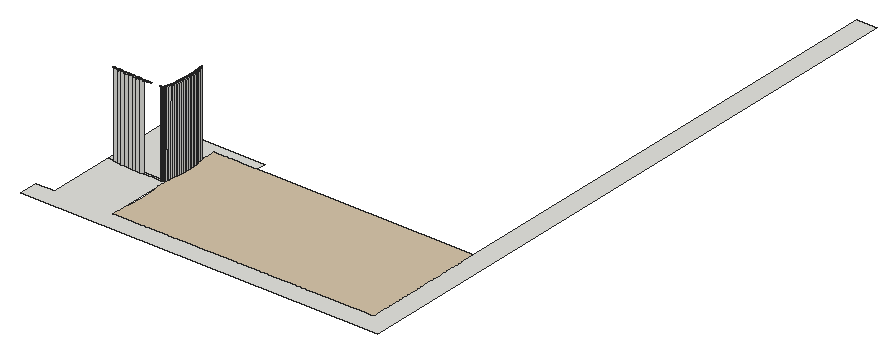
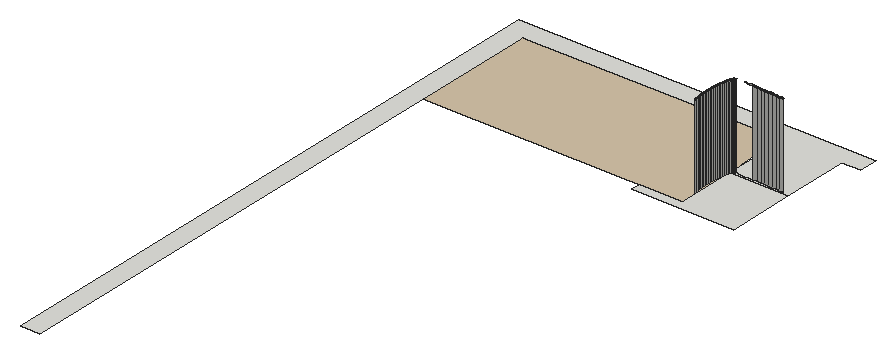
# SketchUp Ruby script. Lengths in inches.
U = 1.inch
M = Sketchup.active_model
def pt(a) = Geom::Point3d.new(a.map { |v| v * U })
def face(e, loops, mat)
  f = e.add_face(loops[0].map { |a| pt(a) })
  loops[1..].each { |l| e.add_face(l.map { |a| pt(a) }).erase! }
  f.material = f.back_material = mat if mat
  f
end
# faces: each face lists its corners as indices into pts; further lists are holes
def faces(e, pts, list, mat = nil) = list.each { |f| face(e, (f[0].is_a?(Array) ? f : [f]).map { |l| l.map { |i| pts[i] } }, mat) }
# xy, xz, yz: faces in a plane at the given z, y or x. An outline is a flat list of corners, or four numbers for a rectangle; further outlines are holes
def ring(l) = l.size == 4 ? [[l[0], l[1]], [l[2], l[1]], [l[2], l[3]], [l[0], l[3]]] : l.each_slice(2).to_a
def flat(e, list, mat, &to3) = list.each { |f| face(e, (f[0].is_a?(Array) ? f : [f]).map { |l| ring(l).map { |u, v| to3.(u, v) } }, mat) }
def xy(e, z, list, mat = nil) = flat(e, list, mat) { |x, y| [x, y, z] }
def xz(e, y, list, mat = nil) = flat(e, list, mat) { |x, z| [x, y, z] }
def yz(e, x, list, mat = nil) = flat(e, list, mat) { |y, z| [x, y, z] }
def lines(e, pts, list) = list.each { |a, b| e.add_line(pt(pts[a]), pt(pts[b])) }
# prism: a flat outline (further loops are holes) pulled along v
def prism(e, loops, v, mat = nil)
  f = face(e, loops, mat); d = Geom::Vector3d.new(v.map { |x| x * U })
  f.pushpull(f.normal.samedirection?(d) ? d.length : -d.length)
end
def box(e, o, s, mat = nil) = prism(e, [[o, [o[0] + s[0], o[1], o[2]], [o[0] + s[0], o[1] + s[1], o[2]], [o[0], o[1] + s[1], o[2]]]], [0, 0, s[2]], mat)
def at(x, y, z, deg = 0) = Geom::Transformation.translation(pt([x, y, z])) * Geom::Transformation.rotation(ORIGIN, Z_AXIS, deg.degrees)
def axes(o, x, y, z) = Geom::Transformation.new([*x, 0, *y, 0, *z, 0, *pt(o).to_a, 1])
def part(name) = M.definitions.add(name)
# library, detail: a bought-in or finely detailed component or shape, given as its bounding box
def library(name, o, s) = part(name).tap { |d| box(d.entities, o, s) }
def detail(e, o, s) = box(e.add_group.entities, o, s)
def put(e, d, t, mat = nil) = e.add_instance(d, t).tap { |i| i.material = mat if mat }
def group(e, t, mat = nil) = e.add_group.tap { |g| g.transformation = t; g.material = mat if mat }.entities
root = M.entities
M.materials.add("[Tile Various Tan]").color = [214, 196, 169]
xy(root,0,[[318.63,38.86,318.63,47.625,327,47.625,327,78.05,328.96,78.05,329,77.96,329.06,77.85,329.13,77.74,329.21,77.65,329.3,77.56,329.4,77.48,329.51,77.41,329.63,77.36,329.75,77.3125,329.87,77.28,330,77.27,331.77,77.16,333.53,77.06,335.3,76.97,337.0625,76.89,338.83,76.82,340.6,76.76,342.37,76.71,344.13,76.67,345.9,76.63,347.67,76.61,349.4375,76.6,351.21,76.59,351.43,76.61,351.64,76.64,351.85,76.71,352.06,76.79,352.25,76.9,352.43,77.03,352.59,77.18,352.73,77.34,352.86,77.53,352.96,77.72,353.04,77.93,353.07,78.05,353.35,78.05,353.35,47.86,471,47.86,471,319.79,480,319.79,480,38.86],[351.21,76.59,349.4375,76.6,347.67,76.61,345.9,76.63,344.13,76.67,342.37,76.71,340.6,76.76,338.83,76.82,337.0625,76.89,335.3,76.97,333.53,77.06,331.77,77.16,330,77.27,329.87,77.28,329.75,77.3125,329.63,77.36,329.51,77.41,329.4,77.48,329.3,77.56,329.21,77.65,329.13,77.74,329.06,77.85,329,77.96,328.96,78.05,353.07,78.05,353.04,77.93,352.96,77.72,352.86,77.53,352.73,77.34,352.59,77.18,352.43,77.03,352.25,76.9,352.06,76.79,351.85,76.71,351.64,76.64,351.43,76.61],[327,78.05,327,108.86,373.1,108.86,373.1,104.36,353.35,104.36,353.35,79.23,353.31,79.03,353.09,78.14,353.07,78.05],[353.07,78.05,353.09,78.14,353.31,79.03,353.35,79.23,353.35,78.05]])
xy(root,0,[[353.35,47.86,353.35,53.98,353.51,54.68,353.69,55.59,353.85,56.5,353.99,57.41,354.12,58.32,354.22,59.24,354.31,60.16,354.375,61.08,354.42,62,354.45,62.92,354.46,63.84,354.45,64.77,354.42,65.6875,354.375,66.61,354.31,67.53,354.22,68.45,354.12,69.36,353.99,70.28,353.85,71.1875,353.69,72.1,353.51,73,353.35,73.7,353.35,79.23,353.51,79.93,353.69,80.84,353.85,81.75,353.99,82.66,354.12,83.57,354.22,84.49,354.31,85.41,354.375,86.33,354.42,87.25,354.45,88.17,354.46,89.09,354.45,90.02,354.42,90.9375,354.375,91.86,354.31,92.78,354.22,93.7,354.12,94.61,353.99,95.53,353.85,96.4375,353.69,97.35,353.51,98.25,353.35,98.95,353.35,104.36,471,104.36,471,47.86],[353.35,79.23,353.35,98.95,353.51,98.25,353.69,97.35,353.85,96.4375,353.99,95.53,354.12,94.61,354.22,93.7,354.31,92.78,354.375,91.86,354.42,90.9375,354.45,90.02,354.46,89.09,354.45,88.17,354.42,87.25,354.375,86.33,354.31,85.41,354.22,84.49,354.12,83.57,353.99,82.66,353.85,81.75,353.69,80.84,353.51,79.93]],"[Tile Various Tan]")
p = [[342.37,76.71,0],[342.37,76.71,37.7],[340.6,76.76,37.7],[340.6,76.76,0],[344.13,76.67,0],[344.13,76.67,37.7],
  [352.06,76.79,0],[352.06,76.79,37.7],[351.85,76.71,37.7],[351.85,76.71,0],[338.83,76.82,0],[338.83,76.82,37.7],
  [337.0625,76.89,37.7],[337.0625,76.89,0],[352.25,76.9,0],[352.25,76.9,37.7],[335.3,76.97,37.7],[335.3,76.97,0],
  [352.43,77.03,0],[352.43,77.03,37.7],[333.53,77.06,37.7],[333.53,77.06,0],[352.59,77.18,0],[352.59,77.18,37.7],
  [331.77,77.16,37.7],[331.77,77.16,0],[330,77.27,37.7],[330,77.27,0],[352.73,77.34,0],[352.73,77.34,37.7],
  [329.87,77.28,37.7],[329.87,77.28,0],[352.86,77.53,0],[352.86,77.53,37.7],[352.96,77.72,0],[352.96,77.72,37.7],
  [353.04,77.93,0],[353.04,77.93,37.7],[353.09,78.14,0],[353.09,78.14,37.7],[353.07,78.05,0],[353.31,79.03,0],
  [353.31,79.03,37.7],[353.51,79.93,0],[353.51,79.93,37.7],[353.35,79.23,0],[353.69,80.84,0],[353.69,80.84,37.7],
  [353.85,81.75,0],[353.85,81.75,37.7],[353.99,82.66,0],[353.99,82.66,37.7],[354.12,83.57,0],[354.12,83.57,37.7],
  [354.22,84.49,0],[354.22,84.49,37.7],[354.31,85.41,0],[354.31,85.41,37.7],[354.375,86.33,0],[354.375,86.33,37.7],
  [354.42,87.25,0],[354.42,87.25,37.7],[354.45,88.17,0],[354.45,88.17,37.7],[354.46,89.09,0],[354.46,89.09,37.7],
  [354.45,90.02,0],[354.45,90.02,37.7],[354.42,90.9375,0],[354.42,90.9375,37.7],[354.375,91.86,0],[354.375,91.86,37.7],
  [354.31,92.78,0],[354.31,92.78,37.7],[354.22,93.7,0],[354.22,93.7,37.7],[354.12,94.61,0],[354.12,94.61,37.7],
  [353.99,95.53,0],[353.99,95.53,37.7],[353.85,96.4375,0],[353.85,96.4375,37.7],[353.69,97.35,0],[353.69,97.35,37.7],
  [342.37,76.71,37.8],[340.6,76.76,37.8],[344.13,76.67,37.8],[352.06,76.79,37.8],[351.85,76.71,37.8],[338.83,76.83,37.8],
  [337.0625,76.9,37.8],[352.25,76.9,37.8],[335.3,76.97,37.8],[352.42,77.03,37.8],[333.53,77.0625,37.8],[352.59,77.18,37.8],
  [331.77,77.16,37.8],[330,77.27,37.8],[352.73,77.35,37.8],[329.875,77.29,37.8],[352.85,77.53,37.8],[352.95,77.72,37.8],
  [353.03,77.93,37.8],[353.09,78.14,37.8],[353.31,79.04,37.8],[353.51,79.9375,37.8],[353.6875,80.84,37.8],[353.85,81.75,37.8],
  [353.99,82.66,37.8],[354.11,83.57,37.8],[354.22,84.49,37.8],[354.31,85.41,37.8],[354.37,86.33,37.8],[354.42,87.25,37.8],
  [354.45,88.17,37.8],[354.46,89.09,37.8],[354.45,90.02,37.8],[354.42,90.9375,37.8],[354.37,91.86,37.8],[354.31,92.78,37.8],
  [354.22,93.7,37.8],[354.11,94.61,37.8],[353.99,95.53,37.8],[353.85,96.4375,37.8],[353.6875,97.35,37.8],[342.37,76.72,37.89],
  [340.6,76.78,37.89],[344.13,76.68,37.89],[352.05,76.8,37.89],[351.85,76.72,37.89],[338.83,76.84,37.89],[337.0625,76.91,37.89],
  [352.24,76.91,37.89],[335.3,76.99,37.89],[352.42,77.04,37.89],[333.53,77.07,37.89],[352.58,77.1875,37.89],[331.77,77.17,37.89],
  [330,77.28,37.89],[352.72,77.35,37.89],[329.875,77.3,37.89],[352.84,77.53,37.89],[352.94,77.73,37.89],[353.02,77.93,37.89],
  [353.08,78.14,37.89],[353.3,79.04,37.89],[353.49,79.9375,37.89],[353.68,80.84,37.89],[353.84,81.75,37.89],[353.98,82.66,37.89],
  [354.1,83.57,37.89],[354.21,84.49,37.89],[354.29,85.41,37.89],[354.36,86.33,37.89],[354.41,87.25,37.89],[354.4375,88.17,37.89],
  [354.45,89.09,37.89],[354.4375,90.01,37.89],[354.41,90.9375,37.89],[354.36,91.86,37.89],[354.29,92.78,37.89],[354.21,93.7,37.89],
  [354.1,94.61,37.89],[353.98,95.52,37.89],[353.84,96.4375,37.89],[353.68,97.34,37.89],[342.37,76.74,37.99],[340.6,76.79,37.99],
  [344.13,76.7,37.99],[351.84,76.74,37.99],[351.64,76.66,37.89],[351.64,76.68,37.99],[352.04,76.82,37.99],[338.83,76.86,37.99],
  [337.07,76.93,37.99],[352.23,76.93,37.99],[335.3,77,37.99],[352.4,77.05,37.99],[333.53,77.09,37.99],[352.5625,77.2,37.99],
  [331.77,77.19,37.99],[330,77.3,37.99],[352.7,77.36,37.99],[329.88,77.31,37.99],[329.75,77.33,37.89],[329.76,77.34,37.99],
  [352.83,77.54,37.99],[352.93,77.73,37.99],[353.01,77.94,37.99],[353.06,78.15,37.99],[353.28,79.04,37.99],[353.48,79.94,37.99],
  [353.66,80.85,37.99],[353.82,81.75,37.99],[353.96,82.66,37.99],[354.09,83.58,37.99],[354.19,84.49,37.99],[354.28,85.41,37.99],
  [354.34,86.33,37.99],[354.39,87.25,37.99],[354.42,88.17,37.99],[354.43,89.09,37.99],[354.42,90.01,37.99],[354.39,90.9375,37.99],
  [354.34,91.86,37.99],[354.28,92.78,37.99],[354.19,93.69,37.99],[354.09,94.61,37.99],[353.96,95.52,37.99],[353.82,96.43,37.99],
  [353.66,97.34,37.99],[342.37,76.77,38.08],[340.6,76.82,38.08],[344.14,76.73,38.08],[345.9,76.69,38.08],[345.9,76.67,37.99],
  [351.83,76.76,38.08],[351.63,76.7,38.08],[352.03,76.84,38.08],[338.83,76.88,38.08],[352.22,76.95,38.08],[337.07,76.95,38.08],
  [335.3,77.03,38.08],[352.39,77.07,38.08],[333.53,77.12,38.08],[331.77,77.22,38.08],[352.55,77.22,38.08],[330.01,77.32,38.08],
  [352.68,77.38,38.08],[329.88,77.34,38.08],[329.77,77.37,38.08],[352.8,77.56,38.08],[352.9,77.74,38.08],[352.98,77.94,38.08],
  [353.03,78.15,38.08],[353.25,79.05,38.08],[353.45,79.95,38.08],[353.63,80.85,38.08],[353.79,81.76,38.08],[353.9375,82.67,38.08],
  [354.06,83.58,38.08],[354.16,84.5,38.08],[354.25,85.41,38.08],[354.32,86.33,38.08],[354.37,87.25,38.08],[354.39,88.17,38.08],
  [354.4,89.09,38.08],[354.39,90.01,38.08],[354.37,90.93,38.08],[354.32,91.85,38.08],[354.25,92.77,38.08],[354.16,93.69,38.08],
  [354.06,94.61,38.08],[353.9375,95.52,38.08],[353.79,96.43,38.08],[353.63,97.34,38.08],[344.14,76.76,38.17],[342.37,76.8,38.17],
  [345.9,76.73,38.17],[347.67,76.7,38.17],[347.67,76.67,38.08],[351.62,76.73,38.17],[351.42,76.66,38.08],[351.42,76.7,38.17],
  [351.82,76.79,38.17],[340.6,76.85,38.17],[338.83,76.91,38.17],[352.02,76.875,38.17],[352.2,76.98,38.17],[337.07,76.98,38.17],
  [352.37,77.1,38.17],[335.3,77.0625,38.17],[333.54,77.15,38.17],[331.77,77.25,38.17],[352.52,77.24,38.17],[330.01,77.36,38.17],
  [352.66,77.4,38.17],[329.89,77.37,38.17],[329.77,77.4,38.17],[352.78,77.57,38.17],[352.875,77.76,38.17],[352.95,77.95,38.17],
  [353,78.16,38.17],[353.22,79.06,38.17],[353.42,79.95,38.17],[353.6,80.86,38.17],[353.76,81.76,38.17],[353.9,82.67,38.17],
  [354.03,83.58,38.17],[354.13,84.5,38.17],[354.22,85.42,38.17],[354.28,86.33,38.17],[354.33,87.25,38.17],[354.36,88.17,38.17],
  [354.37,89.09,38.17],[354.36,90.01,38.17],[354.33,90.93,38.17],[354.28,91.85,38.17],[354.22,92.77,38.17],[354.13,93.6875,38.17],
  [354.03,94.6,38.17],[353.9,95.51,38.17],[353.76,96.42,38.17],[353.6,97.33,38.17]]
faces(root,p,[[0,1,2,3],[4,5,1,0],[6,7,8,9],[10,11,12,13],[3,2,11,10],[14,15,7,6],[13,12,16,17],[18,19,15,14],
  [17,16,20,21],[22,23,19,18],[21,20,24,25],[25,24,26,27],[28,29,23,22],[27,26,30,31],[32,33,29,28],[34,35,33,32],
  [36,37,35,34],[38,39,37,36,40],[41,42,39,38],[43,44,42,41,45],[46,47,44,43],[48,49,47,46],[50,51,49,48],[52,53,51,50],
  [54,55,53,52],[56,57,55,54],[58,59,57,56],[60,61,59,58],[62,63,61,60],[64,65,63,62],[66,67,65,64],[68,69,67,66],
  [70,71,69,68],[72,73,71,70],[74,75,73,72],[76,77,75,74],[78,79,77,76],[80,81,79,78],[82,83,81,80],[84,1,2,85],
  [86,5,1,84],[87,7,8,88],[89,11,12,90],[85,2,11,89],[91,15,7,87],[90,12,16,92],[93,19,15,91],[92,16,20,94],
  [95,23,19,93],[94,20,24,96],[96,24,26,97],[98,29,23,95],[97,26,30,99],[100,33,29,98],[101,35,33,100],[102,37,35,101],
  [103,39,37,102],[104,42,39,103],[105,44,42,104],[106,47,44,105],[107,49,47,106],[108,51,49,107],[109,53,51,108],[110,55,53,109],
  [111,57,55,110],[112,59,57,111],[113,61,59,112],[114,63,61,113],[115,65,63,114],[116,67,65,115],[117,69,67,116],[118,71,69,117],
  [119,73,71,118],[120,75,73,119],[121,77,75,120],[122,79,77,121],[123,81,79,122],[124,83,81,123],[125,84,85,126],[127,86,84,125],
  [128,87,88,129],[130,89,90,131],[126,85,89,130],[132,91,87,128],[131,90,92,133],[134,93,91,132],[133,92,94,135],[136,95,93,134],
  [135,94,96,137],[137,96,97,138],[139,98,95,136],[138,97,99,140],[141,100,98,139],[142,101,100,141],[143,102,101,142],[144,103,102,143],
  [145,104,103,144],[146,105,104,145],[147,106,105,146],[148,107,106,147],[149,108,107,148],[150,109,108,149],[151,110,109,150],[152,111,110,151],
  [153,112,111,152],[154,113,112,153],[155,114,113,154],[156,115,114,155],[157,116,115,156],[158,117,116,157],[159,118,117,158],[160,119,118,159],
  [161,120,119,160],[162,121,120,161],[163,122,121,162],[164,123,122,163],[165,124,123,164],[166,125,126,167],[168,127,125,166],[169,129,170,171],
  [172,128,129,169],[173,130,131,174],[167,126,130,173],[175,132,128,172],[174,131,133,176],[177,134,132,175],[176,133,135,178],[179,136,134,177],
  [178,135,137,180],[180,137,138,181],[182,139,136,179],[183,140,184,185],[181,138,140,183],[186,141,139,182],[187,142,141,186],[188,143,142,187],
  [189,144,143,188],[190,145,144,189],[191,146,145,190],[192,147,146,191],[193,148,147,192],[194,149,148,193],[195,150,149,194],[196,151,150,195],
  [197,152,151,196],[198,153,152,197],[199,154,153,198],[200,155,154,199],[201,156,155,200],[202,157,156,201],[203,158,157,202],[204,159,158,203],
  [205,160,159,204],[206,161,160,205],[207,162,161,206],[208,163,162,207],[209,164,163,208],[210,165,164,209],[211,166,167,212],[213,168,166,211],
  [214,215,168,213],[216,169,171,217],[218,172,169,216],[212,167,173,219],[220,175,172,218],[221,174,176,222],[219,173,174,221],[223,177,175,220],
  [222,176,178,224],[224,178,180,225],[226,179,177,223],[225,180,181,227],[228,182,179,226],[229,183,185,230],[227,181,183,229],[231,186,182,228],
  [232,187,186,231],[233,188,187,232],[234,189,188,233],[235,190,189,234],[236,191,190,235],[237,192,191,236],[238,193,192,237],[239,194,193,238],
  [240,195,194,239],[241,196,195,240],[242,197,196,241],[243,198,197,242],[244,199,198,243],[245,200,199,244],[246,201,200,245],[247,202,201,246],
  [248,203,202,247],[249,204,203,248],[250,205,204,249],[251,206,205,250],[252,207,206,251],[253,208,207,252],[254,209,208,253],[255,210,209,254],
  [256,213,211,257],[258,214,213,256],[259,260,214,258],[261,217,262,263],[264,216,217,261],[265,212,219,266],[257,211,212,265],[267,218,216,264],
  [268,220,218,267],[266,219,221,269],[270,223,220,268],[271,222,224,272],[269,221,222,271],[272,224,225,273],[274,226,223,270],[273,225,227,275],
  [276,228,226,274],[277,229,230,278],[275,227,229,277],[279,231,228,276],[280,232,231,279],[281,233,232,280],[282,234,233,281],[283,235,234,282],
  [284,236,235,283],[285,237,236,284],[286,238,237,285],[287,239,238,286],[288,240,239,287],[289,241,240,288],[290,242,241,289],[291,243,242,290],
  [292,244,243,291],[293,245,244,292],[294,246,245,293],[295,247,246,294],[296,248,247,295],[297,249,248,296],[298,250,249,297],[299,251,250,298],
  [300,252,251,299],[301,253,252,300],[302,254,253,301],[303,255,254,302]])
